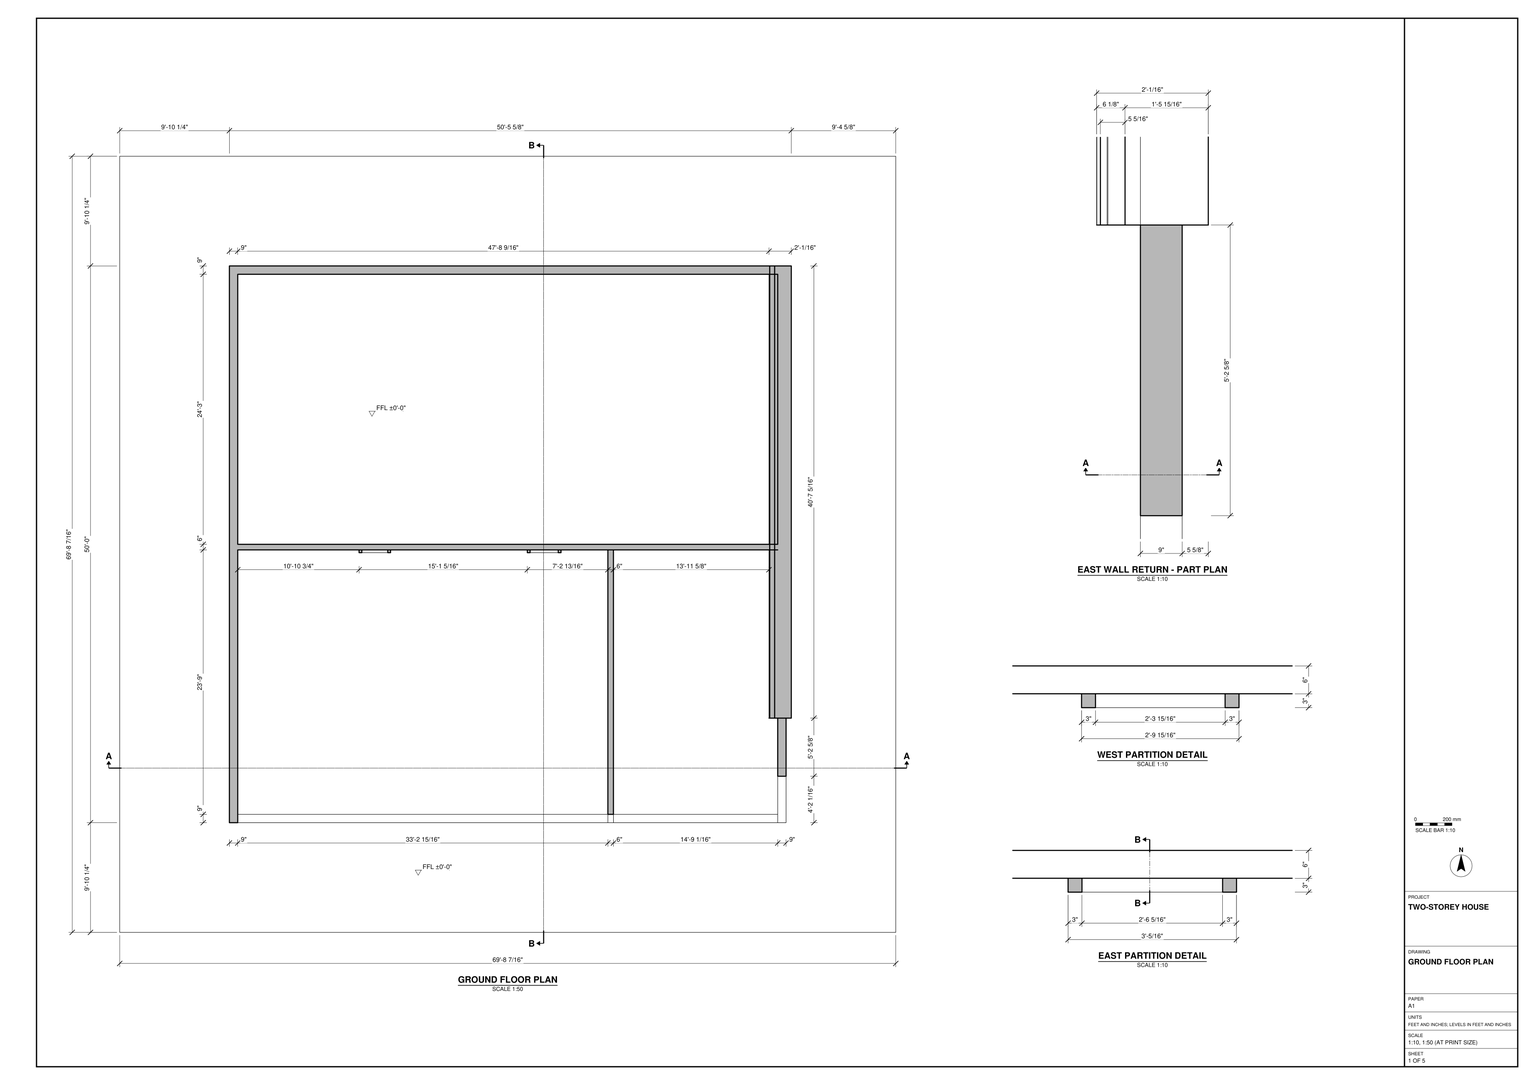
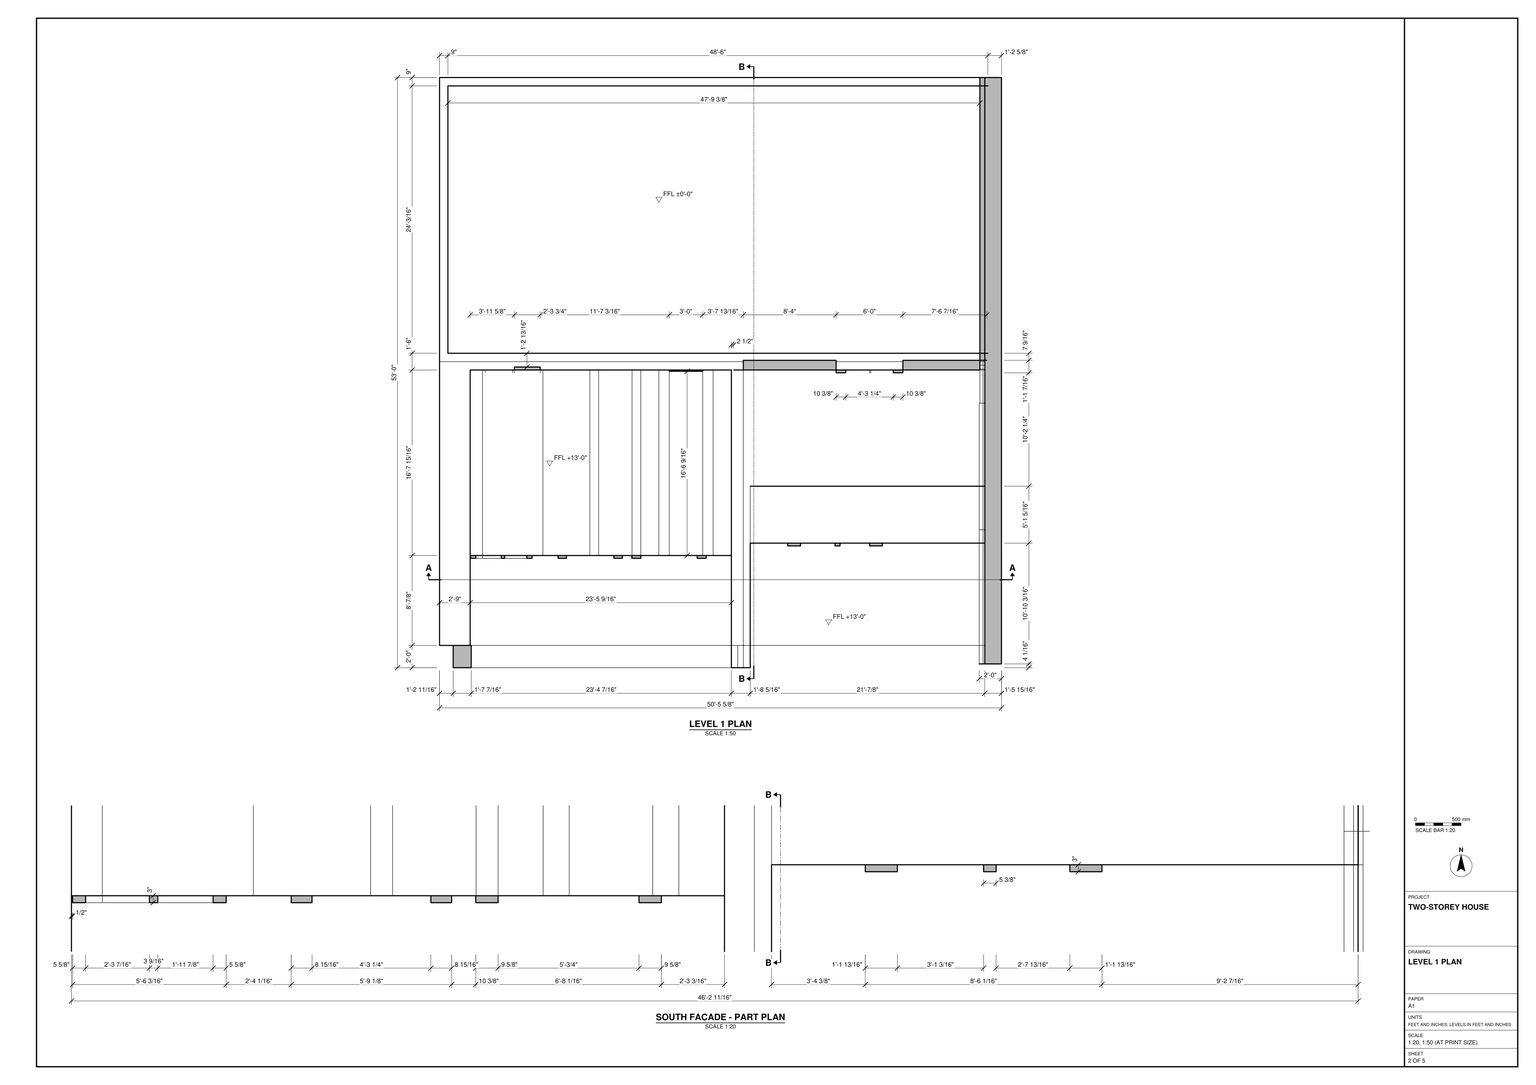
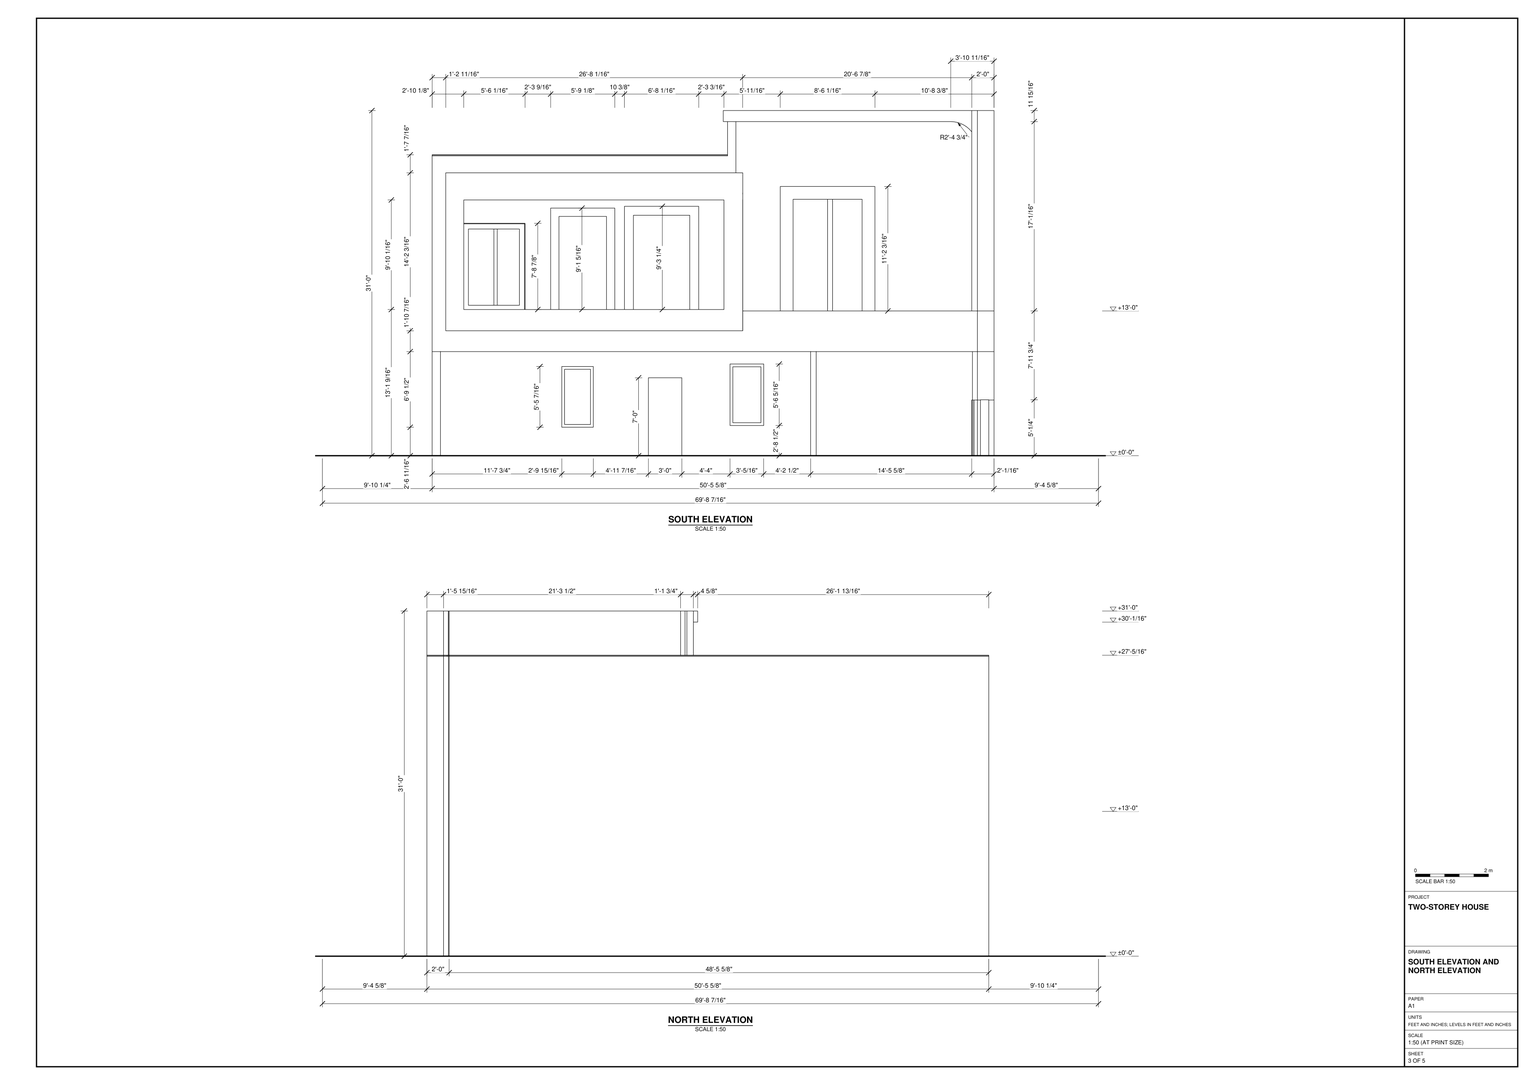
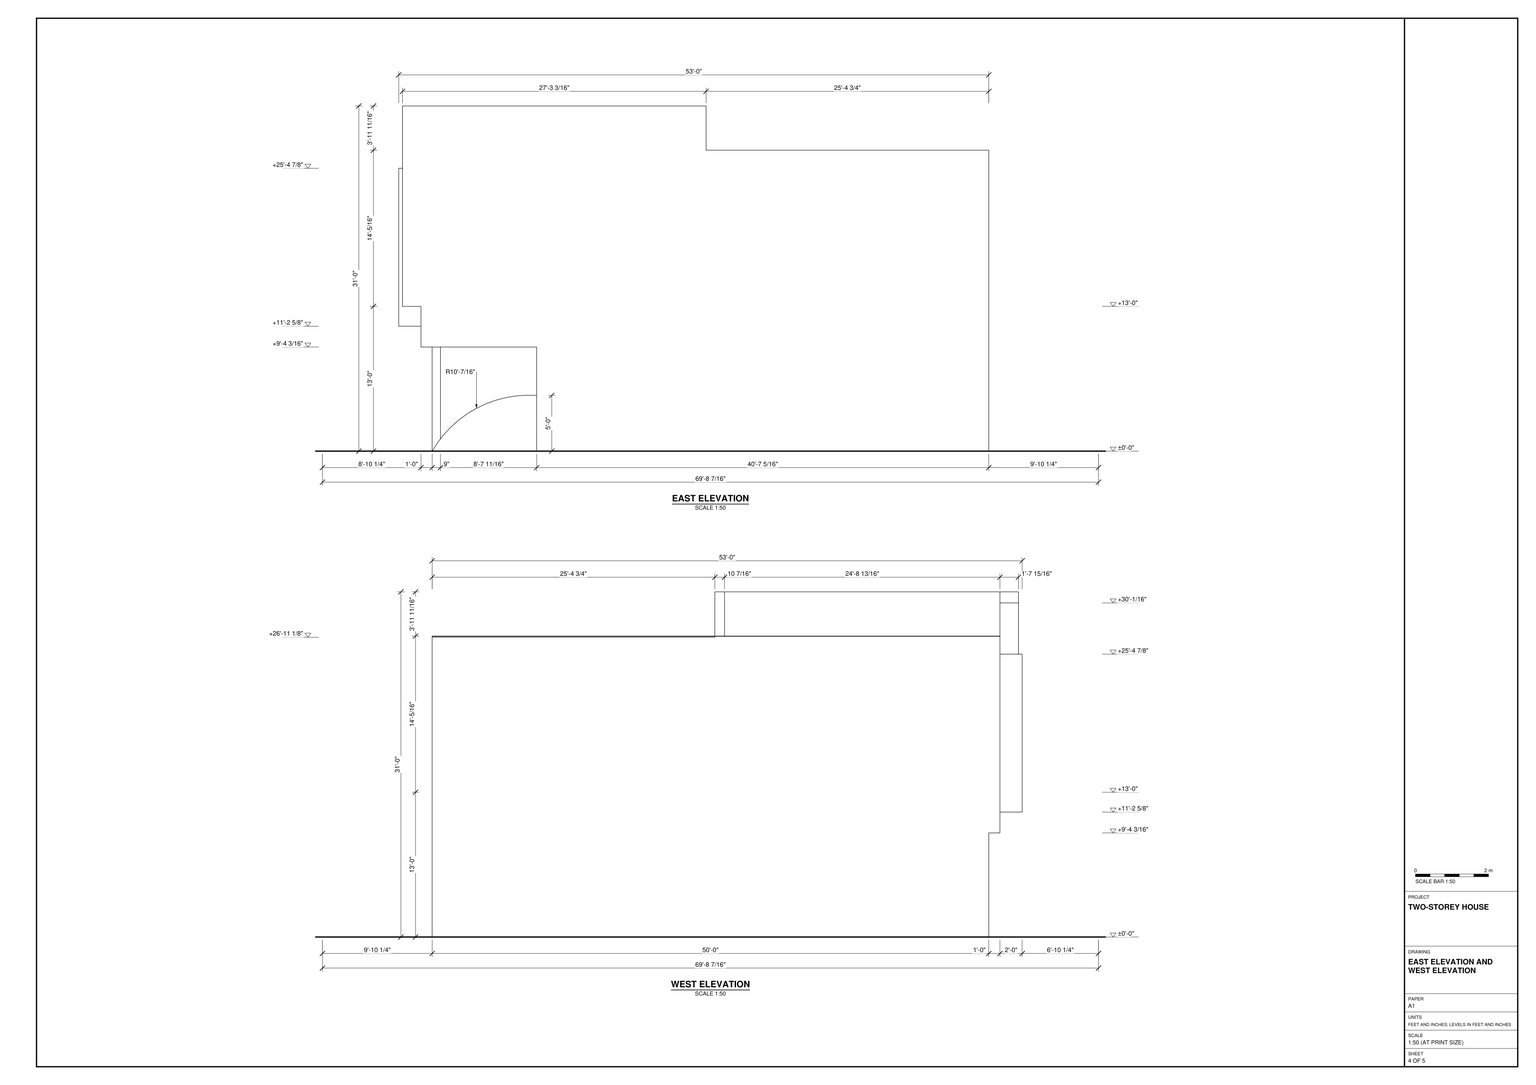
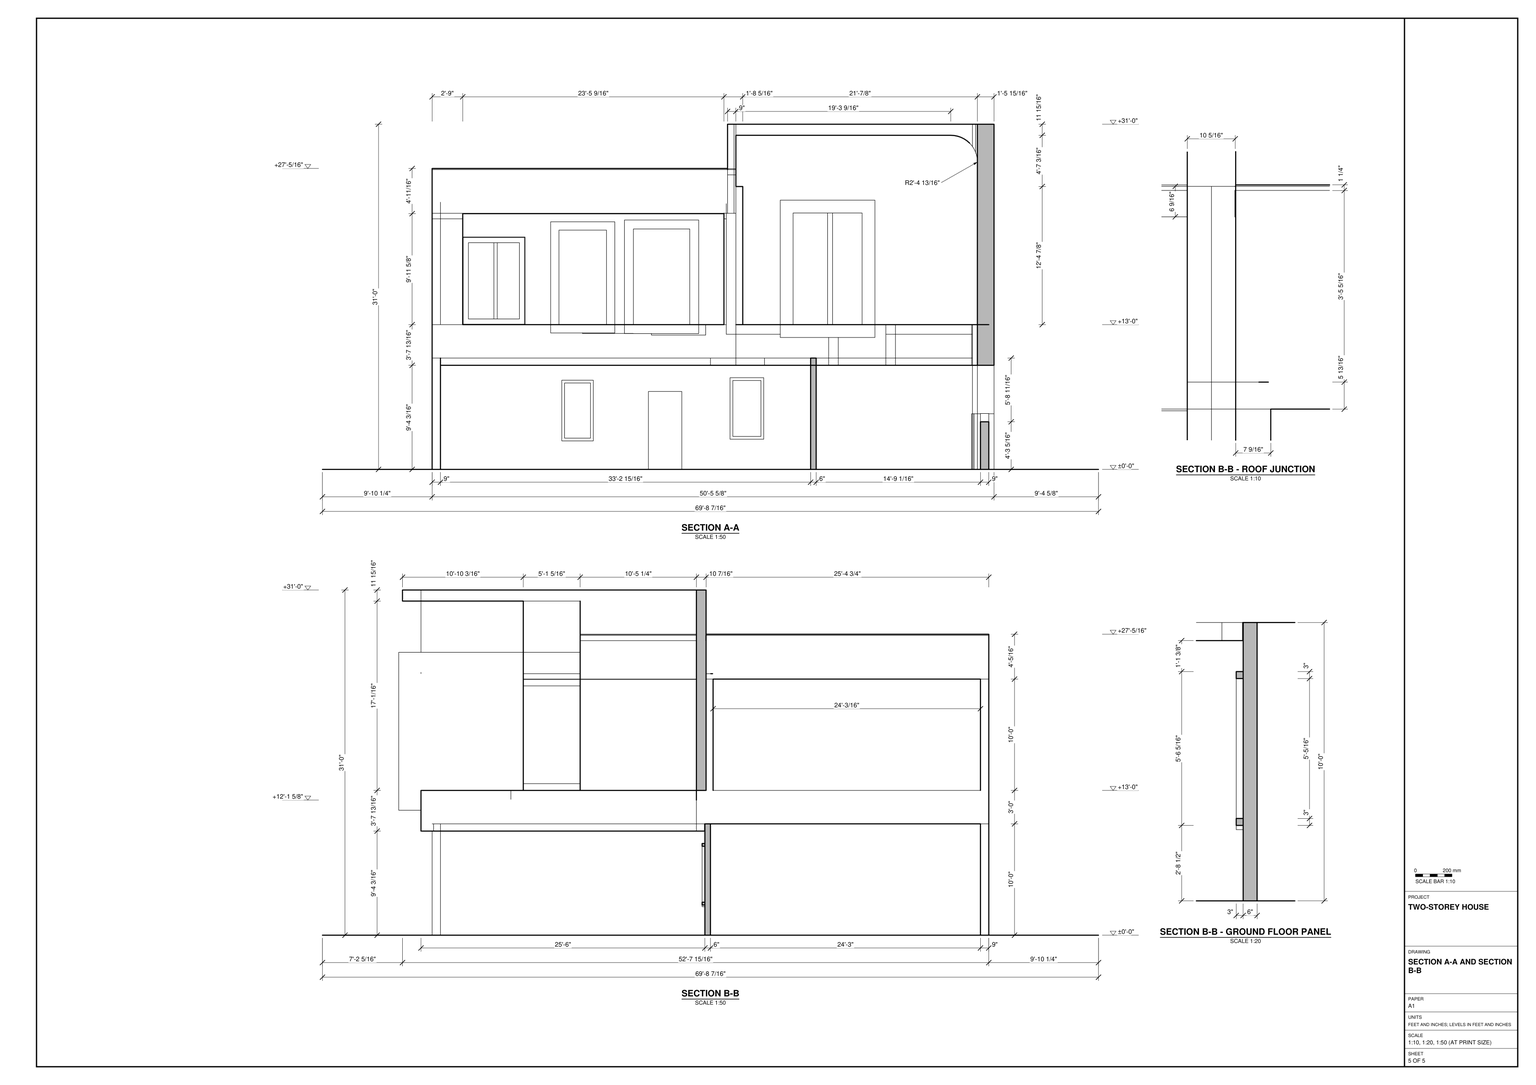
Build the house in SketchUp from task_files/diagram_01.pdf. Work in feet and inches. Include the square site plane: the overall model measures 69'-8 7/16" east to west by 69'-8 7/16" north to south and is 31'-0" high. Set the ground floor at ±0'-0" and the upper floor at +13'-0".

Locate the house on the site using the setbacks on the ground floor plan. Model the perimeter walls, the large rear enclosure and the partition that divides the front into a wider west bay and a narrower east bay. Follow the wall thicknesses as drawn, including the east wall return. Use the upper floor plan and the elevations together to establish the slab edges, facade projections and roof profile. On the south side, place the ground floor doorway between the windows. Above them, build the projecting rectangular surround on the west and the higher canopy on the east, including its curved junction with the end wall.

Keep walls, slabs and roof elements in separate groups or components. Group any furniture or joinery shown by piece and use components for repeated parts. Any decor or loose items shown may be suitable library components. Save one SketchUp model as output_files/two_storey_house_with_its_stepped_south_facade.skp.

# SketchUp Ruby script. Lengths in inches.
U = 1.inch
M = Sketchup.active_model
def pt(a) = Geom::Point3d.new(a.map { |v| v * U })
def face(e, loops, mat)
  f = e.add_face(loops[0].map { |a| pt(a) })
  loops[1..].each { |l| e.add_face(l.map { |a| pt(a) }).erase! }
  f.material = f.back_material = mat if mat
  f
end
# faces: each face lists its corners as indices into pts; further lists are holes
def faces(e, pts, list, mat = nil) = list.each { |f| face(e, (f[0].is_a?(Array) ? f : [f]).map { |l| l.map { |i| pts[i] } }, mat) }
# xy, xz, yz: faces in a plane at the given z, y or x. An outline is a flat list of corners, or four numbers for a rectangle; further outlines are holes
def ring(l) = l.size == 4 ? [[l[0], l[1]], [l[2], l[1]], [l[2], l[3]], [l[0], l[3]]] : l.each_slice(2).to_a
def flat(e, list, mat, &to3) = list.each { |f| face(e, (f[0].is_a?(Array) ? f : [f]).map { |l| ring(l).map { |u, v| to3.(u, v) } }, mat) }
def xy(e, z, list, mat = nil) = flat(e, list, mat) { |x, y| [x, y, z] }
def xz(e, y, list, mat = nil) = flat(e, list, mat) { |x, z| [x, y, z] }
def yz(e, x, list, mat = nil) = flat(e, list, mat) { |y, z| [x, y, z] }
def lines(e, pts, list) = list.each { |a, b| e.add_line(pt(pts[a]), pt(pts[b])) }
# prism: a flat outline (further loops are holes) pulled along v
def prism(e, loops, v, mat = nil)
  f = face(e, loops, mat); d = Geom::Vector3d.new(v.map { |x| x * U })
  f.pushpull(f.normal.samedirection?(d) ? d.length : -d.length)
end
def box(e, o, s, mat = nil) = prism(e, [[o, [o[0] + s[0], o[1], o[2]], [o[0] + s[0], o[1] + s[1], o[2]], [o[0], o[1] + s[1], o[2]]]], [0, 0, s[2]], mat)
def at(x, y, z, deg = 0) = Geom::Transformation.translation(pt([x, y, z])) * Geom::Transformation.rotation(ORIGIN, Z_AXIS, deg.degrees)
def axes(o, x, y, z) = Geom::Transformation.new([*x, 0, *y, 0, *z, 0, *pt(o).to_a, 1])
def part(name) = M.definitions.add(name)
# library, detail: a bought-in or finely detailed component or shape, given as its bounding box
def library(name, o, s) = part(name).tap { |d| box(d.entities, o, s) }
def detail(e, o, s) = box(e.add_group.entities, o, s)
def put(e, d, t, mat = nil) = e.add_instance(d, t).tap { |i| i.material = mat if mat }
def group(e, t, mat = nil) = e.add_group.tap { |g| g.transformation = t; g.material = mat if mat }.entities
root = M.entities
xy(root,0,[[[0,0,836.45,836.45],[118.22,118.22,118.22,718.22,723.85,718.22,723.85,230.91,718.22,230.91,718.22,118.22]],[118.22,118.22,118.22,718.22,699.79,718.22,699.79,709.22,127.22,709.22,127.22,418.22,699.79,418.22,699.79,412.22,127.22,412.22,127.22,118.22],[127.22,118.22,526.16,127.22],[526.16,118.22,532.16,127.22],[532.16,118.22,709.22,127.22],
  [709.22,118.22,718.22,230.91],[127.22,127.22,526.16,412.22],[526.16,127.22,532.16,412.22],[532.16,127.22,709.22,127.22,709.22,230.91,699.79,230.91,699.79,412.22,532.16,412.22],[699.79,230.91,699.85,412.22],
  [699.85,230.91,700.6,412.22],[700.6,230.91,702.04,412.22],[702.04,230.91,702.22,412.22],[702.22,230.91,705.91,412.22],[705.91,230.91,709.22,412.22],
  [709.22,230.91,723.85,412.22],[699.79,412.22,699.85,418.22],[699.85,412.22,700.6,418.22],[700.6,412.22,702.04,418.22],[702.04,412.22,702.22,418.22],
  [702.22,412.22,705.91,418.22],[705.91,412.22,723.85,418.22],[127.22,418.22,699.79,709.22],[699.79,418.22,699.85,709.22],[699.85,418.22,700.6,709.22],
  [700.6,418.22,702.04,709.22],[702.04,418.22,702.22,709.22],[702.22,418.22,705.91,709.22],[705.91,418.22,709.22,709.22],[709.22,418.22,723.85,709.22],
  [699.79,709.22,699.85,718.22],[699.85,709.22,700.6,718.22],[700.6,709.22,702.04,718.22],[702.04,709.22,702.22,718.22],[702.22,709.22,705.91,718.22],
  [705.91,709.22,723.85,718.22]])
xy(root,30.7,[[257.99,409.22,291.92,412.22]])
xy(root,32.53,[[439.33,409.22,475.64,412.22]])
xy(root,33.7,[[260.99,409.22,288.92,412.22]])
xy(root,35.53,[[442.33,409.22,472.64,412.22]])
xy(root,93.13,[[260.99,409.22,288.92,412.22]])
xy(root,95.84,[[442.33,409.22,472.64,412.22]])
xy(root,96.13,[[257.99,409.22,291.92,412.22]])
xy(root,98.84,[[439.33,409.22,475.64,412.22]])
xy(root,112.1875,[[118.22,106.22,118.22,118.22,127.22,118.22,127.22,412.06,709.22,412.06,709.22,403.93,700.6,403.93,700.6,230.91,705.91,230.91,705.91,106.22],[705.91,106.22,723.85,230.91],[700.6,230.91,702.22,367.31],[702.22,230.91,709.22,367.31],[700.6,367.31,702.22,403.06],
  [700.6,403.06,702.22,403.93],[702.22,403.06,709.22,403.93]])
xy(root,120,[[526.16,127.22,532.16,412.06],[703.97,403.06,708.04,403.93],[708.04,403.06,709.22,403.93],[709.22,403.06,717.97,403.93],[127.22,412.06,418.22,412.22],
  [418.22,412.06,476.45,412.22],[476.45,412.06,526.16,412.22],[526.16,412.06,532.16,412.22],[532.16,412.06,709.22,412.22],[127.22,412.22,418.22,418.22],
  [418.22,412.22,476.45,418.22],[476.45,412.22,709.22,418.22],[127.22,418.22,418.22,709.22],[418.22,418.22,476.45,709.22],[476.45,418.22,709.22,709.22]])
xy(root,134.64,[[132.9,82.22,452.97,106.22]])
xy(root,156,[[699.85,86.29,703.97,106.22],[703.97,86.29,705.73,106.22],[705.73,86.29,705.91,106.22],[705.91,86.29,705.97,106.22],[705.97,86.29,717.97,106.22],
  [717.97,86.29,723.85,106.22],[151.22,106.22,432.76,106.22,432.76,203.12,405.55,203.12,405.55,200.12,395.91,200.12,395.91,203.12,335.16,203.12,335.16,200.12,325.52,200.12,325.52,203.12,315.125,203.12,315.125,200.12,306.17,200.12,306.17,203.12,254.92,203.12,254.92,200.12,245.97,200.12,245.97,203.12,151.22,203.12],[445.64,106.22,453.05,106.22,453.05,277.79,699.85,277.79,699.85,367.31,700.6,367.31,700.6,403.06,617.62,403.06,617.62,400.06,607.24,400.06,607.24,403.06,583.0625,403.06,583.0625,400.06,581.62,400.06,581.62,403.06,556,403.06,556,400.06,545.62,400.06,545.62,403.06,445.64,403.06],[453.05,106.22,699.85,106.22,699.85,216.47,595.49,216.47,595.49,213.47,581.66,213.47,581.66,216.47,549.84,216.47,549.84,213.47,544.47,213.47,544.47,216.47,507.28,216.47,507.28,213.47,493.45,213.47,493.45,216.47,453.05,216.47],[699.85,106.22,703.97,216.47],
  [703.97,106.22,705.97,216.47],[705.97,106.22,708.04,216.47],[708.04,106.22,717.97,230.91],[717.97,106.22,718.22,230.91],[245.97,200.12,254.92,203.12],
  [306.17,200.12,315.125,203.12],[325.52,200.12,325.68,203.12],[325.68,200.12,335.16,203.12],[395.91,200.12,401.83,203.12],[401.83,200.12,405.55,203.12],
  [151.22,203.12,164.53,403.06],[164.53,203.12,229.65,403.06],[229.65,203.12,280.19,403.06],[280.19,203.12,289.68,403.06],[289.68,203.12,325.68,403.06],
  [325.68,203.12,335.16,403.06],[335.16,203.12,354.58,403.06],[354.58,203.12,365.83,403.06],[365.83,203.12,401.83,401.68],[401.83,203.12,413.07,403.06],
  [413.07,203.12,432.76,403.06],[493.45,213.47,507.28,216.47],[544.47,213.47,549.84,216.47],[581.66,213.47,595.49,216.47],[453.05,216.47,699.85,277.79],
  [699.85,216.47,703.97,230.91],[703.97,216.47,705.97,230.91],[705.97,216.47,708.04,230.91],[699.85,230.91,703.97,277.79],[703.97,230.91,705.97,277.79],
  [705.97,230.91,708.04,277.79],[699.85,277.79,703.97,367.31],[703.97,277.79,705.97,367.31],[700.6,367.31,703.97,403.06],[703.97,367.31,705.97,403.06],
  [705.97,367.31,708.04,403.06],[545.62,400.06,556,403.06],[581.62,400.06,583.0625,403.06],[607.24,400.06,617.62,403.06],[365.83,401.68,401.83,403.06],
  [445.64,403.06,545.62,408.28],[617.62,403.06,700.6,408.28],[700.6,403.06,705.97,403.93],[700.6,403.93,703.97,408.28],[703.97,403.93,705.97,408.28],
  [705.97,403.93,708.04,408.28],[445.64,408.28,545.62,412.06],[617.62,408.28,700.6,412.06],[700.6,408.28,703.97,412.06],[703.97,408.28,705.97,412.06],
  [705.97,408.28,708.04,412.06],[445.64,412.06,545.62,413.5],[617.62,412.06,700.6,413.5],[700.6,412.06,703.97,413.5],[703.97,412.06,705.97,413.5],
  [705.97,412.06,708.04,413.5]])
xy(root,156.5,[[151.73,200.12,164.53,203.12],[164.53,200.12,217.91,203.12]])
xy(root,157.54,[[152.35,82.22,432.76,106.22]])
xy(root,159,[[198.875,403.06,226.65,406.25]])
xy(root,162.125,[[157.35,200.12,164.53,203.12],[164.53,200.12,184.82,203.12],[184.82,200.12,188.41,203.12],[188.41,200.12,212.29,203.12]])
xy(root,229.625,[[556,400.06,581.62,403.06],[581.62,400.06,583.0625,403.06],[583.0625,400.06,607.24,403.06]])
xy(root,240,[[545.62,400.06,617.62,403.06],[365.83,401.68,401.83,403.06],[545.62,403.06,617.62,408.28],[545.62,408.28,617.62,413.5]])
xy(root,244.3125,[[157.35,200.12,184.82,203.12],[184.82,200.12,188.41,203.12],[188.41,200.12,212.29,203.12]])
xy(root,249.93,[[151.73,200.12,217.91,203.12]])
xy(root,257.875,[[254.92,200.12,306.17,203.12]])
xy(root,258.375,[[198.875,403.06,226.65,406.25]])
xy(root,259.125,[[335.16,200.12,395.91,203.12]])
xy(root,266.83,[[245.97,200.12,315.125,203.12]])
xy(root,268.77,[[325.52,200.12,405.55,203.12]])
xy(root,275.625,[[152.35,82.22,152.35,106.22,151.22,106.22,151.22,203.12,432.76,203.12,432.76,82.22],[151.22,203.12,432.76,403.06]])
xy(root,276,[[127.22,421.06,709.22,709.22]])
xy(root,276.34,[[507.28,213.47,544.47,216.47],[544.47,213.47,549.84,216.47],[549.84,213.47,581.66,216.47]])
xy(root,281.8125,[[445.64,418.5,700.6,420.54]])
xy(root,290.17,[[493.45,213.47,595.49,216.47]])
xy(root,304.86,[[132.9,82.22,453.05,106.22],[445.64,106.22,453.05,216.47]])
xy(root,323.125,[[700.6,403.06,700.79,408.28],[700.6,408.28,700.79,412.06],[699.79,412.06,700.6,412.15],[700.6,412.06,700.79,412.15],[699.79,412.15,699.79,413.5,450.39,413.5,450.39,413.43],
  [699.79,412.15,700.6,413.5],[700.6,412.15,700.79,413.5],[699.79,413.5,700.6,718.22],[700.6,413.5,702.22,718.22]])
xy(root,324,[[436.64,403.06,436.64,413.5,443.64,413.46,443.64,403.06],[698.1,408.28,700.6,412.06],[700.6,412.15,450.39,413.43,700.6,413.43],[450.39,413.43,450.39,413.46,445.64,413.46,445.64,413.45],[450.39,413.43,700.6,413.46],
  [445.64,413.45,445.64,413.46,443.64,413.46],[443.64,413.46,443.64,413.5,436.64,413.5],[443.64,413.46,445.64,413.5],[445.64,413.46,450.39,413.5],[450.39,413.46,700.6,413.5]])
xy(root,324.3125,[[118.22,106.22,436.64,106.22,436.64,413.5,699.85,413.5,699.85,718.22,118.22,718.22],[700.6,403.06,700.79,408.28],[700.79,403.06,703.97,408.28],[703.97,403.06,708.04,408.28],[700.6,408.28,700.79,413.5],
  [700.79,408.28,703.97,413.5],[703.97,408.28,708.04,413.5],[699.85,413.5,700.6,718.22],[700.6,413.5,705.91,718.22],[705.91,413.5,723.85,718.22]])
xy(root,360.08,[[432.01,86.29,432.01,106.22,445.64,106.22,445.64,216.47,677.17,216.47,677.17,86.29]])
xy(root,372,[[432.01,86.29,699.85,86.29,699.85,403.06,436.64,403.06,436.64,106.22,432.01,106.22],[699.85,86.29,705.91,106.22],[705.91,86.29,717.97,106.22],[717.97,86.29,723.85,106.22],[699.85,106.22,705.91,403.06],
  [705.91,106.22,717.97,403.06],[717.97,106.22,723.85,106.22,723.85,413.5,705.91,413.5,705.91,403.06,717.97,403.06],[436.64,403.06,445.64,413.5],[445.64,403.06,699.85,413.5],[699.85,403.06,700.6,413.5],
  [700.6,403.06,705.91,413.5]])
xz(root,82.22,[[[132.9,134.64,452.97,134.64,452.97,276,453.05,276,453.05,304.86,132.9,304.86],[152.35,157.54,432.76,275.625]],[452.97,134.64,453.05,156],[452.97,156,453.05,276]])
xz(root,86.29,[[699.85,156,705.91,372],[705.91,156,723.85,372],[699.85,349.01,699.85,372,432.01,372,432.01,360.08,677.17,360.08,680.93,359.83,684.63,359.1,688.2,357.89,691.57,356.22,694.71,354.125,697.54,351.64]])
xz(root,106.22,[[118.22,112.1875,705.91,112.1875,705.91,156,453.05,156,453.05,134.64,132.9,134.64,132.9,304.86,445.64,304.86,445.64,360.08,436.64,360.08,436.64,323.125,118.22,323.125],[705.91,112.1875,723.85,156],[132.9,134.64,132.9,304.86,445.64,304.86,445.64,298.35,140.22,298.35,140.22,141.97,445.64,141.97,445.64,134.64],[445.64,134.64,445.72,141.97],[445.72,134.64,452.97,145.6875],
  [452.97,134.64,453.05,156],[140.22,141.97,152.35,141.97,152.35,156,151.22,156,151.22,276,140.22,276],[152.35,141.97,152.35,153.16,439.64,153.16,439.64,145.6875,445.64,145.6875,445.64,141.97],[445.64,141.97,445.72,145.6875],[439.64,145.6875,445.64,156],
  [445.64,145.6875,445.72,156],[445.72,145.6875,452.97,156],[152.35,153.16,439.64,156],[151.22,156,152.35,275.625],[152.35,156,432.76,157.54],
  [432.76,156,445.64,157.54],[445.64,156,445.72,157.54],[445.64,157.54,445.72,163.33],[445.64,163.33,445.72,268.67],[445.64,268.67,445.72,281.8125],
  [140.22,276,145.04,298.35],[445.64,281.8125,445.72,298.35],[118.22,324,436.64,324.3125],[432.01,360.08,436.64,372]])
xz(root,118.22,[[118.22,0,127.22,112.1875]])
xz(root,127.22,[[526.16,0,532.16,120]])
xz(root,200.12,[[245.97,156,254.92,156,254.92,257.875,306.17,257.875,306.17,156,315.125,156,315.125,266.83,245.97,266.83],[325.52,156,335.16,156,335.16,259.125,395.91,259.125,395.91,156,405.55,156,405.55,268.77,325.52,268.77],[[151.73,156.5,217.91,249.93],[157.35,162.125,212.29,244.3125]],[184.82,162.125,188.41,244.3125]])
xz(root,203.12,[[325.52,146.36,405.55,156],[245.97,147.05,315.125,156],[218.41,156,245.97,156,245.97,266.83,315.125,266.83,315.125,156,325.52,156,325.52,268.77,405.55,268.77,405.55,156,432.76,156,432.76,275.625,151.22,275.625,151.22,250.4375,218.41,250.4375],[[151.22,156,218.41,250.4375],[151.73,156.5,217.91,249.93]],[245.97,156,245.97,266.83,315.125,266.83,315.125,156,306.17,156,306.17,257.875,254.92,257.875,254.92,156],
  [254.92,156,306.17,257.875],[325.52,156,325.52,268.77,405.55,268.77,405.55,156,395.91,156,395.91,259.125,335.16,259.125,335.16,156],[335.16,156,395.91,259.125],[[151.73,156.5,217.91,249.93],[157.35,162.125,212.29,244.3125]],[157.35,162.125,184.82,244.3125],
  [184.82,162.125,188.41,244.3125],[188.41,162.125,212.29,244.3125]])
xz(root,213.47,[[493.45,156,507.28,156,507.28,276.34,581.66,276.34,581.66,156,595.49,156,595.49,290.17,493.45,290.17],[544.47,156,549.84,276.34]])
xz(root,216.47,[[493.45,142.17,595.49,156],[453.05,156,493.45,156,493.45,290.17,595.49,290.17,595.49,156,705.97,156,705.97,331.28,705.73,335.04,704.99,338.73,703.78,342.3,702.12,345.68,700.02,348.81,697.54,351.64,694.71,354.125,691.57,356.22,688.2,357.89,684.63,359.1,680.93,359.83,677.17,360.08,445.64,360.08,445.64,304.86,453.05,304.86],[493.45,156,493.45,290.17,595.49,290.17,595.49,156,581.66,156,581.66,276.34,507.28,276.34,507.28,156],[507.28,156,544.47,276.34],[544.47,156,549.84,276.34],
  [549.84,156,581.66,276.34]])
xz(root,230.91,[[699.79,0,699.85,60],[699.85,0,700.6,60],[700.6,0,702.04,60],[702.04,0,702.22,60],[702.22,0,705.91,60],
  [705.91,0,709.22,60],[709.22,0,718.22,60],[718.22,0,723.85,60],[700.6,60,705.91,112.1875],[705.91,60,723.85,112.1875],
  [709.22,112.1875,718.22,120],[709.1,120,709.22,156]])
xz(root,277.79,[[453.05,156,453.05,304.86,445.64,304.86,445.64,360.08,677.17,360.08,680.93,359.83,684.63,359.1,688.2,357.89,691.57,356.22,694.71,354.125,697.54,351.64,700.02,348.81,702.12,345.68,703.78,342.3,704.99,338.73,705.73,335.04,705.97,331.28,705.97,156]])
xz(root,367.31,[[700.6,112.1875,709.22,156]])
xz(root,400.06,[[545.62,156,556,156,556,229.625,607.24,229.625,607.24,156,617.62,156,617.62,240,545.62,240]])
xz(root,401.68,[[365.83,156,401.83,240]])
xz(root,403.06,[[700.6,112.1875,700.6,145.625,703.97,145.625,703.97,120,709.22,120,709.22,112.1875],[703.97,120,708.04,145.625],[354.58,144.75,413.07,156],[435.26,145.625,445.64,276],[445.64,145.625,545.62,156],
  [545.62,145.625,556,156],[617.62,145.625,700.6,156],[700.6,145.625,703.97,156],[703.97,145.625,708.04,156],[280.19,146.52,335.16,156],
  [151.22,156,151.22,275.625,432.76,275.625,432.76,156,413.07,156,413.07,251.25,354.58,251.25,354.58,156,335.16,156,335.16,249.48,280.19,249.48,280.19,156,229.65,156,229.65,261.375,164.53,261.375,164.53,156],[[164.53,156,229.65,261.375],[167.53,159,226.65,258.375]],[280.19,156,280.19,249.48,335.16,249.48,335.16,156,325.68,156,325.68,240,289.68,240,289.68,156],[289.68,156,325.68,240],[354.58,156,354.58,251.25,413.07,251.25,413.07,156,401.83,156,401.83,240,365.83,240,365.83,156],
  [365.83,156,401.83,240],[445.64,156,545.62,156,545.62,240,617.62,240,617.62,156,700.6,156,700.6,372,445.64,372],[545.62,156,545.62,240,617.62,240,617.62,156,607.24,156,607.24,229.625,556,229.625,556,156],[556,156,581.62,229.625],[581.62,156,583.0625,229.625],
  [583.0625,156,607.24,229.625],[167.53,159,197.09,258.375],[197.09,159,198.875,258.375],[198.875,159,226.65,258.375],[151.22,275.625,432.76,276],
  [700.6,322.5625,700.79,323.125],[700.6,323.125,700.72,324.3125],[700.72,323.125,700.79,324.3125],[436.64,324,443.64,372],[443.64,324,445.64,372],
  [700.6,324.3125,703.97,372],[703.97,324.3125,708.04,372]])
xz(root,403.93,[[700.6,112.1875,709.22,112.1875,709.22,120,703.97,120,703.97,156,700.6,156],[703.97,120,708.04,156]])
xz(root,406.25,[[198.875,159,226.65,258.375]])
xz(root,409.22,[[[257.99,30.7,291.92,96.13],[260.99,33.7,288.92,93.13]],[[439.33,32.53,475.64,98.84],[442.33,35.53,472.64,95.84]]])
xz(root,412.06,[[127.22,112.1875,418.22,120],[418.22,112.1875,476.45,120],[476.45,112.1875,709.22,120],[700.79,322.1875,702.22,322.5625],[698.1,322.5625,700.79,323.125],
  [698.1,323.125,699.79,324]])
xz(root,412.22,[[[127.22,0,351.35,0,351.35,84,387.35,84,387.35,0,526.16,0,526.16,120,127.22,120],[439.33,32.53,475.64,98.84],[257.99,30.7,291.92,96.13]],[351.35,0,387.35,84],[526.16,0,532.16,120],[532.16,0,709.22,120],[[257.99,30.7,291.92,96.13],[260.99,33.7,288.92,93.13]],
  [[439.33,32.53,475.64,98.84],[442.33,35.53,472.64,95.84]],[260.99,33.7,288.92,93.13],[442.33,35.53,472.64,95.84]])
xz(root,413.5,[[445.64,156,445.64,270.0625,699.79,270.0625,699.79,323.125,700.6,323.125,700.6,156,617.62,156,617.62,240,545.62,240,545.62,156],[700.6,156,703.97,276],[703.97,156,708.04,276],[436.64,270.0625,443.64,317.4375],[443.64,270.0625,445.64,317.4375],
  [445.64,270.0625,450.39,317.4375],[450.39,270.0625,699.79,323.125],[700.6,276,703.97,281.8125],[703.97,276,708.04,281.8125],[700.6,281.8125,703.97,323.125],
  [703.97,281.8125,708.04,323.125],[436.64,317.4375,443.64,323.125],[443.64,317.4375,445.64,323.125],[445.64,317.4375,450.39,323.125],[436.64,323.125,443.64,324],
  [443.64,323.125,445.64,324],[445.64,323.125,450.39,324],[450.39,323.125,700.6,324],[700.6,323.125,700.79,324],[700.79,323.125,703.97,324],
  [703.97,323.125,708.04,324],[708.04,323.125,717.97,324],[436.64,324,443.64,324.3125],[443.64,324,445.64,324.3125],[445.64,324,450.39,324.3125],
  [450.39,324,700.6,324.3125],[700.6,324,700.79,324.3125],[700.79,324,703.97,324.3125],[703.97,324,708.04,324.3125],[708.04,324,717.97,324.3125],
  [436.64,324.3125,443.64,372],[443.64,324.3125,445.64,372],[445.64,324.3125,450.39,372],[450.39,324.3125,699.85,372],[699.85,324.3125,700.6,372],
  [700.6,324.3125,700.79,372],[700.79,324.3125,705.91,372],[705.91,324.3125,723.85,372]])
xz(root,418.22,[[127.22,0,709.22,120]])
xz(root,421.06,[[127.22,156,709.22,276]])
xz(root,709.22,[[127.22,0,709.22,120],[127.22,156,709.22,276]])
xz(root,718.22,[[118.22,0,699.85,323.125],[699.85,0,700.6,323.125],[700.6,0,705.91,323.125],[705.91,0,723.85,323.125],[118.22,323.125,699.85,324],
  [699.85,323.125,700.6,324],[700.6,323.125,702.04,324],[702.04,323.125,705.91,324],[705.91,323.125,723.85,324],[118.22,324,699.85,324.3125],
  [699.85,324,700.6,324.3125],[700.6,324,702.04,324.3125],[702.04,324,705.91,324.3125],[705.91,324,723.85,324.3125]])
yz(root,118.22,[[118.22,0,118.22,112.1875,106.22,112.1875,106.22,324,413.5,324,413.5,323.125,718.22,323.125,718.22,0],[106.22,324,413.5,324.3125],[413.5,324,718.22,324.3125]])
yz(root,127.22,[[118.22,0,127.22,112.1875],[127.22,0,412.22,0,412.22,120,412.06,120,412.06,112.1875,127.22,112.1875],[418.22,0,709.22,120],[119.83,112.1875,127.22,120],[127.22,112.1875,412.06,120],
  [421.06,156,709.22,276]])
yz(root,132.9,[[82.22,134.64,106.22,304.86]])
yz(root,151.22,[[106.22,156,203.12,275.625],[203.12,156,403.06,275.625]])
yz(root,151.73,[[200.12,156.5,203.12,249.93]])
yz(root,152.35,[[82.22,157.54,106.22,275.625]])
yz(root,157.35,[[200.12,162.125,203.12,244.3125]])
yz(root,184.82,[[200.12,162.125,203.12,244.3125]])
yz(root,188.41,[[200.12,162.125,203.12,244.3125]])
yz(root,198.875,[[403.06,159,406.25,258.375]])
yz(root,212.29,[[200.12,162.125,203.12,244.3125]])
yz(root,217.91,[[200.12,156.5,203.12,249.93]])
yz(root,226.65,[[403.06,159,406.25,258.375]])
yz(root,245.97,[[200.12,156,203.12,266.83]])
yz(root,254.92,[[200.12,156,203.12,257.875]])
yz(root,257.99,[[409.22,30.7,412.22,96.13]])
yz(root,260.99,[[409.22,33.7,412.22,93.13]])
yz(root,288.92,[[409.22,33.7,412.22,93.13]])
yz(root,291.92,[[409.22,30.7,412.22,96.13]])
yz(root,306.17,[[200.12,156,203.12,257.875]])
yz(root,315.125,[[200.12,156,203.12,266.83]])
yz(root,325.52,[[200.12,156,203.12,268.77]])
yz(root,335.16,[[200.12,156,203.12,259.125]])
yz(root,365.83,[[401.68,156,403.06,240]])
yz(root,395.91,[[200.12,156,203.12,259.125]])
yz(root,401.83,[[401.68,156,403.06,240]])
yz(root,405.55,[[200.12,156,203.12,268.77]])
yz(root,432.01,[[86.29,360.08,106.22,372]])
yz(root,432.76,[[106.22,156,106.22,157.54,82.22,157.54,82.22,275.625,203.12,275.625,203.12,156],[203.12,156,403.06,275.625],[106.22,275.625,403.06,276]])
yz(root,436.64,[[403.06,317.4375,413.5,323.125],[106.22,323.125,403.06,324],[403.06,323.125,413.5,324],[106.22,324,403.06,324.3125],[403.06,324,413.5,324.3125],
  [106.22,324.3125,403.06,372],[403.06,324.3125,413.5,372]])
yz(root,439.33,[[409.22,32.53,412.22,98.84]])
yz(root,442.33,[[409.22,35.53,412.22,95.84]])
yz(root,445.64,[[403.06,156,408.28,276],[408.28,156,413.5,276],[403.06,276,408.28,281.8125],[408.28,276,413.5,281.8125],[403.06,281.8125,408.28,324],
  [408.28,281.8125,413.5,324],[106.22,304.86,216.47,360.08],[216.47,304.86,277.79,360.08],[403.06,324,413.5,372]])
yz(root,450.39,[[413.43,317.4375,413.46,323.125],[413.46,317.4375,413.5,323.125],[413.43,323.125,413.46,324],[413.46,323.125,413.5,324]])
yz(root,453.05,[[82.22,134.64,106.22,134.64,106.22,156,216.47,156,216.47,304.86,82.22,304.86]])
yz(root,472.64,[[409.22,35.53,412.22,95.84]])
yz(root,475.64,[[409.22,32.53,412.22,98.84]])
yz(root,493.45,[[213.47,156,216.47,290.17]])
yz(root,507.28,[[213.47,156,216.47,276.34]])
yz(root,526.16,[[127.22,0,412.22,120]])
yz(root,532.16,[[127.22,0,412.22,120]])
yz(root,544.47,[[213.47,156,216.47,276.34]])
yz(root,545.62,[[400.06,156,403.06,240],[403.06,156,408.28,240],[408.28,156,413.5,240]])
yz(root,549.84,[[213.47,156,216.47,276.34]])
yz(root,556,[[400.06,156,403.06,229.625]])
yz(root,581.66,[[213.47,156,216.47,276.34]])
yz(root,595.49,[[213.47,156,216.47,290.17]])
yz(root,607.24,[[400.06,156,403.06,229.625]])
yz(root,617.62,[[400.06,156,403.06,240],[403.06,156,408.28,240],[408.28,156,413.5,240]])
yz(root,699.79,[[412.15,311.4375,413.5,317.4375],[412.15,317.4375,413.5,323.125]])
yz(root,700.6,[[230.91,0,230.91,112.1875,403.93,112.1875,403.93,156,413.5,156,413.5,281.8125,718.22,281.8125,718.22,0],[367.31,112.1875,403.06,156],[403.06,112.1875,403.93,156],[403.06,156,403.93,276],[403.93,156,408.28,276],
  [408.28,156,413.5,276],[403.06,276,403.93,281.8125],[403.93,276,408.28,281.8125],[408.28,276,413.5,281.8125],[403.06,281.8125,408.28,323.125],
  [408.28,281.8125,413.5,323.125],[403.06,323.125,408.28,324],[408.28,323.125,413.5,324],[413.5,323.125,718.22,324.3125],[403.06,324,413.5,324.3125],
  [403.06,324.3125,413.5,372]])
yz(root,700.79,[[403.06,322.1875,412.06,322.5625],[403.06,322.5625,412.06,323.125],[403.06,323.125,413.5,324.3125]])
yz(root,705.91,[[230.91,0,230.91,112.1875,106.22,112.1875,106.22,156,86.29,156,86.29,372,413.5,372,413.5,324.3125,718.22,324.3125,718.22,0]])
yz(root,705.97,[[216.47,156,277.79,331.28]])
yz(root,709.22,[[118.22,0,124.27,9.4375,131.16,18.27,138.85,26.43,147.26,33.84,156.33,40.43,165.97,46.15,176.09,50.96,186.625,54.8,197.46,57.64,208.52,59.47,219.7,60.25,230.91,60,230.91,0],[418.22,0,709.22,120],[230.91,112.1875,367.31,120],[403.06,112.1875,403.93,120],[403.93,112.1875,412.06,120]])
yz(root,718.22,[[118.22,0,230.91,0,230.91,60,219.7,60.25,208.52,59.47,197.46,57.64,186.625,54.8,176.09,50.96,165.97,46.15,156.33,40.43,147.26,33.84,138.85,26.43,131.16,18.27,124.27,9.4375]])
yz(root,723.85,[[230.91,0,718.22,0,718.22,324.3125,413.5,324.3125,413.5,372,86.29,372,86.29,156,106.22,156,106.22,112.1875,230.91,112.1875]])
p = [[718.22,118.22,0],[718.22,124.27,9.4375],[709.22,124.27,9.4375],[709.22,118.22,0],[718.22,131.16,18.27],[709.22,131.16,18.27],
  [718.22,138.85,26.43],[709.22,138.85,26.43],[718.22,147.26,33.84],[709.22,147.26,33.84],[718.22,156.33,40.43],[709.22,156.33,40.43],
  [718.22,165.97,46.15],[709.22,165.97,46.15],[718.22,176.09,50.96],[709.22,176.09,50.96],[718.22,186.625,54.8],[709.22,186.625,54.8],
  [718.22,197.46,57.64],[709.22,197.46,57.64],[718.22,208.52,59.47],[709.22,208.52,59.47],[718.22,219.7,60.25],[709.22,219.7,60.25],
  [718.22,230.91,60],[709.22,230.91,60],[699.79,412.15,323.125],[450.39,413.43,323.125],[450.39,413.43,317.4375],[699.79,412.15,317.4375],
  [705.97,277.79,331.28],[705.73,277.79,335.04],[705.73,216.47,335.04],[705.97,216.47,331.28],[704.99,277.79,338.73],[704.99,216.47,338.73],
  [697.54,216.47,351.64],[697.54,86.29,351.64],[694.71,86.29,354.125],[694.71,216.47,354.125],[691.57,86.29,356.22],[691.57,216.47,356.22],
  [688.2,86.29,357.89],[688.2,216.47,357.89],[684.63,86.29,359.1],[684.63,216.47,359.1],[680.93,86.29,359.83],[680.93,216.47,359.83],
  [677.17,86.29,360.08],[677.17,216.47,360.08],[718.22,135.34,9],[709.22,135.34,9],[127.22,127.22,120],[118.22,127.22,120],
  [127.22,412.06,120],[118.22,412.06,120],[118.22,412.06,156],[445.64,412.06,156],[709.22,412.06,120],[718.22,412.06,120],
  [476.45,709.22,120],[476.45,718.22,120],[709.22,709.22,120],[709.22,718.22,120],[418.22,709.22,120],[418.22,718.22,120],
  [127.22,709.22,120],[127.22,718.22,120],[127.22,119.83,120],[127.22,118.22,120],[127.22,403.06,276],[127.22,403.06,288],
  [127.22,403.31,276],[127.22,403.31,288],[127.22,421.06,276],[127.22,709.22,276],[127.22,718.22,276],[709.22,709.22,276],
  [718.22,709.22,276],[118.22,709.22,276],[151.22,403.06,276],[453.05,106.22,163.33],[445.72,106.22,163.33],[445.72,106.22,268.67],
  [453.05,106.22,268.67],[140.22,106.22,141.97],[140.22,82.22,141.97],[445.72,106.22,157.54],[445.72,82.22,157.54],[445.64,106.22,163.33],
  [439.64,106.22,163.33],[445.64,106.22,268.67],[439.64,106.22,268.67],[439.64,106.22,145.6875],[439.64,82.22,145.6875],[445.72,106.22,145.6875],
  [445.72,82.22,145.6875],[445.72,106.22,141.97],[445.72,82.22,141.97],[152.35,106.22,141.97],[152.35,82.22,141.97],[439.64,106.22,156],
  [439.64,82.22,156],[152.35,106.22,153.16],[152.35,82.22,153.16],[439.64,106.22,153.16],[439.64,82.22,153.16],[140.22,106.22,276],
  [140.22,82.22,276],[145.04,106.22,276],[145.04,82.22,276],[145.04,106.22,298.35],[145.04,82.22,298.35],[445.64,106.22,276],
  [432.76,106.22,276],[435.26,403.06,286.375],[435.26,403.06,276],[607.24,403.06,145.625],[617.62,403.06,145.625],[432.76,403.06,276],
  [452.97,106.22,281.8125],[453.05,106.22,281.8125],[445.72,106.22,281.8125],[452.97,106.22,283.33],[445.64,418.5,281.8125],[445.64,413.5,281.8125],
  [699.97,408.28,324],[699.97,408.28,324.3125],[700.6,408.28,324.3125],[450.39,413.43,324],[450.39,403.06,324],[545.62,412.06,156],
  [617.62,412.06,156],[699.79,718.22,317.4375],[699.79,413.5,317.4375],[436.64,106.22,317.4375],[436.64,403.06,317.4375],[699.79,412.15,311.4375],
  [702.22,412.14,311.4375],[436.64,413.5,270.0625],[118.22,413.5,270.0625],[699.79,718.22,270.0625],[699.79,413.5,270.0625],[699.97,403.06,324.3125],
  [709.22,367.31,120],[709.22,403.06,120],[607.24,403.06,156],[617.62,403.06,112.1875],[607.24,403.06,112.1875],[556,403.06,145.625],
  [556,403.06,112.1875],[545.62,403.06,145.625],[545.62,403.06,112.1875],[445.64,403.06,145.625],[445.64,403.06,112.1875],[716.29,230.91,120],
  [716.29,230.91,156],[716.29,106.22,120],[698.1,403.06,324],[698.1,408.28,324],[698.1,412.06,322.5625],[698.1,403.06,322.5625],
  [698.1,412.06,324],[691.54,412.06,324],[700.6,408.28,324],[700.79,408.28,324],[700.6,412.15,324],[700.79,412.15,324],
  [700.6,413.43,324],[700.79,413.43,324],[718.22,412.14,323.125],[700.79,412.14,323.125],[700.6,408.28,276],[718.22,408.28,276],
  [718.22,403.93,281.8125],[700.6,403.93,281.8125],[718.22,408.28,281.8125],[700.6,408.28,281.8125],[700.6,420.54,281.8125],[718.22,420.54,281.8125],
  [700.79,106.22,323.125],[700.6,106.22,323.125],[708.04,403.06,324.3125],[718.22,403.06,324.3125],[717.97,413.5,323.125],[718.22,413.5,323.125],
  [705.97,413.5,156],[705.97,421.06,156],[705.97,430.91,156],[445.64,106.22,360.08],[445.64,106.22,372],[197.09,403.06,159],
  [197.09,400.06,159],[167.53,403.06,159],[167.53,400.06,159],[197.09,403.06,258.375],[197.09,400.06,258.375],[167.53,403.06,258.375],
  [167.53,400.06,258.375],[198.875,403.06,258.375],[198.875,400.06,258.375],[226.65,403.06,258.375],[226.65,400.06,258.375],[198.875,403.06,159],
  [198.875,400.06,159],[226.65,403.06,159],[226.65,400.06,159],[164.53,403.06,261.375],[164.53,400.06,261.375],[229.65,403.06,261.375],
  [229.65,400.06,261.375],[280.19,403.06,249.48],[280.19,400.06,249.48],[335.16,403.06,249.48],[335.16,400.06,249.48],[354.58,403.06,251.25],
  [354.58,400.06,251.25],[413.07,403.06,251.25],[413.07,400.06,251.25],[325.68,403.06,240],[325.68,400.06,240],[289.68,403.06,240],
  [289.68,400.06,240],[401.83,401.68,240],[401.83,400.06,240],[365.83,401.68,240],[365.83,400.06,240],[703.78,277.79,342.3],
  [703.78,216.47,342.3],[702.12,277.79,345.68],[702.12,216.47,345.68],[700.02,277.79,348.81],[700.02,216.47,348.81],[697.54,277.79,351.64],
  [694.71,277.79,354.125],[691.57,277.79,356.22],[688.2,277.79,357.89],[684.63,277.79,359.1],[680.93,277.79,359.83],[453.05,277.79,304.86],
  [453.05,216.47,304.86],[677.17,277.79,360.08],[453.05,277.79,281.8125],[453.05,216.47,281.8125],[453.05,277.79,268.67],[453.05,216.47,268.67],
  [453.05,277.79,163.33],[453.05,216.47,163.33],[703.97,106.22,372],[703.97,106.22,156],[718.22,413.5,281.8125],[716.29,413.5,281.8125],
  [718.22,413.5,276],[716.29,413.5,276],[717.97,403.06,145.625],[710.98,403.06,145.625],[709.22,413.5,281.8125],[708.04,413.5,281.8125],
  [709.22,413.5,276],[708.04,413.5,276],[709.22,412.06,156],[708.04,412.06,156],[709.22,403.93,156],[708.04,403.93,156],
  [709.22,403.06,145.625],[708.04,403.06,145.625],[708.04,106.22,372],[708.04,106.22,156],[699.85,367.31,156],[699.85,367.31,112.1875],
  [718.22,367.31,156],[709.22,367.31,156]]
faces(root,p,[[0,1,2,3],[1,4,5,2],[4,6,7,5],[6,8,9,7],[8,10,11,9],[10,12,13,11],[12,14,15,13],[14,16,17,15],
  [16,18,19,17],[18,20,21,19],[20,22,23,21],[22,24,25,23],[26,27,28,29],[30,31,32,33],[31,34,35,32],[36,37,38,39],
  [39,38,40,41],[41,40,42,43],[43,42,44,45],[45,44,46,47],[47,46,48,49]])
lines(root,p,[[50,51],[52,53],[54,55],[56,57],[58,59],[60,61],[62,63],[64,65],[66,67],[68,69],[70,71],[72,73],
  [72,74],[75,76],[77,78],[75,79],[72,70],[70,80],[81,82],[83,84],[85,86],[87,88],[89,90],[91,92],
  [93,94],[95,96],[97,98],[99,100],[101,102],[103,104],[105,106],[107,108],[109,110],[111,112],[113,114],[115,116],
  [117,118],[116,119],[120,121],[120,122],[120,123],[124,125],[126,127],[128,127],[129,130],[131,132],[133,134],[135,136],
  [137,138],[139,140],[141,142],[143,127],[144,145],[146,117],[118,147],[117,148],[149,150],[151,152],[153,154],[155,156],
  [155,157],[158,159],[160,161],[162,163],[164,165],[166,167],[168,169],[170,171],[172,173],[174,175],[176,177],[178,179],
  [180,181],[182,183],[184,185],[186,187],[187,188],[189,190],[191,192],[193,194],[195,196],[197,198],[199,200],[201,202],
  [203,204],[205,206],[207,208],[209,210],[211,212],[213,214],[215,216],[217,218],[219,220],[221,222],[223,224],[225,226],
  [227,228],[229,230],[231,232],[233,36],[234,39],[235,41],[236,43],[237,45],[238,47],[239,240],[241,49],[242,243],
  [244,245],[246,247],[248,249],[250,251],[252,253],[254,255],[256,257],[251,256],[258,259],[253,258],[260,261],[262,263],
  [264,265],[255,264],[266,267],[268,269],[270,271]])
